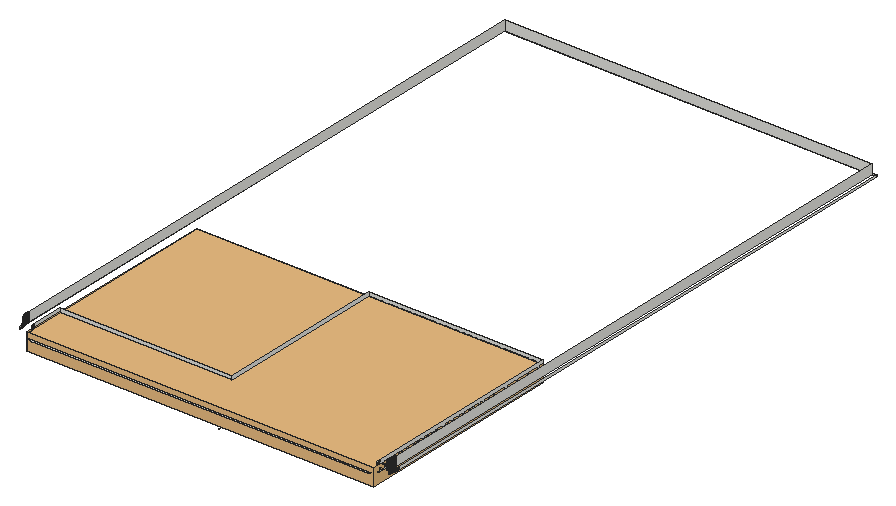
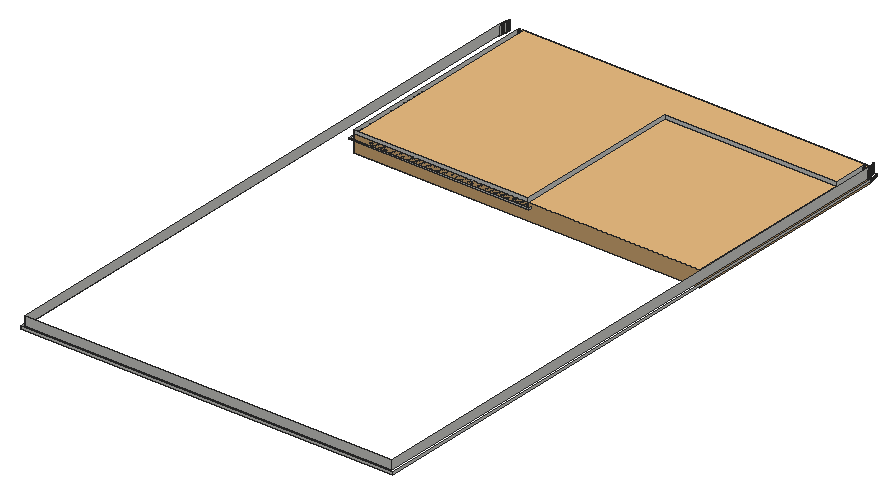
# SketchUp Ruby script. Lengths in inches.
U = 1.inch
M = Sketchup.active_model
def pt(a) = Geom::Point3d.new(a.map { |v| v * U })
def face(e, loops, mat)
  f = e.add_face(loops[0].map { |a| pt(a) })
  loops[1..].each { |l| e.add_face(l.map { |a| pt(a) }).erase! }
  f.material = f.back_material = mat if mat
  f
end
# faces: each face lists its corners as indices into pts; further lists are holes
def faces(e, pts, list, mat = nil) = list.each { |f| face(e, (f[0].is_a?(Array) ? f : [f]).map { |l| l.map { |i| pts[i] } }, mat) }
# xy, xz, yz: faces in a plane at the given z, y or x. An outline is a flat list of corners, or four numbers for a rectangle; further outlines are holes
def ring(l) = l.size == 4 ? [[l[0], l[1]], [l[2], l[1]], [l[2], l[3]], [l[0], l[3]]] : l.each_slice(2).to_a
def flat(e, list, mat, &to3) = list.each { |f| face(e, (f[0].is_a?(Array) ? f : [f]).map { |l| ring(l).map { |u, v| to3.(u, v) } }, mat) }
def xy(e, z, list, mat = nil) = flat(e, list, mat) { |x, y| [x, y, z] }
def xz(e, y, list, mat = nil) = flat(e, list, mat) { |x, z| [x, y, z] }
def yz(e, x, list, mat = nil) = flat(e, list, mat) { |y, z| [x, y, z] }
def lines(e, pts, list) = list.each { |a, b| e.add_line(pt(pts[a]), pt(pts[b])) }
# prism: a flat outline (further loops are holes) pulled along v
def prism(e, loops, v, mat = nil)
  f = face(e, loops, mat); d = Geom::Vector3d.new(v.map { |x| x * U })
  f.pushpull(f.normal.samedirection?(d) ? d.length : -d.length)
end
def box(e, o, s, mat = nil) = prism(e, [[o, [o[0] + s[0], o[1], o[2]], [o[0] + s[0], o[1] + s[1], o[2]], [o[0], o[1] + s[1], o[2]]]], [0, 0, s[2]], mat)
def at(x, y, z, deg = 0) = Geom::Transformation.translation(pt([x, y, z])) * Geom::Transformation.rotation(ORIGIN, Z_AXIS, deg.degrees)
def axes(o, x, y, z) = Geom::Transformation.new([*x, 0, *y, 0, *z, 0, *pt(o).to_a, 1])
def part(name) = M.definitions.add(name)
# library, detail: a bought-in or finely detailed component or shape, given as its bounding box
def library(name, o, s) = part(name).tap { |d| box(d.entities, o, s) }
def detail(e, o, s) = box(e.add_group.entities, o, s)
def put(e, d, t, mat = nil) = e.add_instance(d, t).tap { |i| i.material = mat if mat }
def group(e, t, mat = nil) = e.add_group.tap { |g| g.transformation = t; g.material = mat if mat }.entities
root = M.entities
M.materials.add("Material \#1").color = [140, 140, 140]
c1 = library("Group\#25",[0,0,-11.0625],[292.45,179,14.0625])
xy(root,75.82,[[138.95,197.84,138.95,197.86,138.89,197.86],[138.95,197.84,139.01,197.84,139.01,197.86],[138.95,197.84,139.01,197.86,138.95,197.86],[139.01,197.84,139.0625,197.88,139.01,197.86],[139.01,197.84,139.07,197.86,139.0625,197.88],
  [138.89,197.86,138.9,197.88,138.84,197.9],[138.89,197.86,138.95,197.86,138.9,197.88],[139.07,197.86,139.1,197.91,139.0625,197.88],[139.07,197.86,139.12,197.9,139.1,197.91],[138.9,197.88,138.86,197.91,138.84,197.9],
  [138.84,197.9,138.86,197.91,138.81,197.95],[139.12,197.9,139.13,197.96,139.1,197.91],[139.12,197.9,139.15,197.95,139.13,197.96],[138.86,197.91,138.83,197.96,138.81,197.95],[138.81,197.95,138.83,197.96,138.8,198.01],
  [139.15,197.95,139.14,198.01,139.13,197.96],[139.15,197.95,139.16,198.01,139.14,198.01],[138.83,197.96,138.82,198.01,138.8,198.01],[138.8,198.01,138.82,198.01,138.81,198.07],[138.82,198.01,138.83,198.0625,138.81,198.07],
  [139.14,198.01,139.16,198.01,139.13,198.0625],[139.16,198.01,139.15,198.07,139.13,198.0625],[138.83,198.0625,138.84,198.12,138.81,198.07],[138.83,198.0625,138.86,198.11,138.84,198.12],[139.13,198.0625,139.15,198.07,139.1,198.11],
  [139.15,198.07,139.12,198.12,139.1,198.11],[138.86,198.11,138.89,198.15,138.84,198.12],[138.86,198.11,138.9,198.14,138.89,198.15],[139.1,198.11,139.12,198.12,139.0625,198.14],[139.12,198.12,139.07,198.15,139.0625,198.14],
  [138.9,198.14,138.95,198.17,138.89,198.15],[138.9,198.14,138.95,198.16,138.95,198.17],[139.0625,198.14,139.07,198.15,139.01,198.16],[139.07,198.15,139.01,198.17,139.01,198.16],[138.95,198.16,139.01,198.16,139.01,198.17],
  [138.95,198.16,139.01,198.17,138.95,198.17]],"Material \#1")
xy(root,75.84,[[138.95,197.84,138.89,197.86,138.9,197.88],[138.95,197.84,138.9,197.88,138.95,197.86],[138.95,197.84,138.95,197.86,139.01,197.84],[139.01,197.84,138.95,197.86,139.01,197.86],[139.01,197.84,139.01,197.86,139.07,197.86],
  [138.89,197.86,138.84,197.9,138.86,197.91],[138.89,197.86,138.86,197.91,138.9,197.88],[139.01,197.86,139.0625,197.88,139.07,197.86],[139.07,197.86,139.0625,197.88,139.12,197.9],[139.0625,197.88,139.1,197.91,139.12,197.9],
  [138.84,197.9,138.81,197.95,138.83,197.96],[138.84,197.9,138.83,197.96,138.86,197.91],[139.12,197.9,139.1,197.91,139.15,197.95],[139.1,197.91,139.13,197.96,139.15,197.95],[138.81,197.95,138.8,198.01,138.82,198.01],
  [138.81,197.95,138.82,198.01,138.83,197.96],[139.15,197.95,139.13,197.96,139.16,198.01],[139.13,197.96,139.14,198.01,139.16,198.01],[138.8,198.01,138.81,198.07,138.83,198.0625],[138.8,198.01,138.83,198.0625,138.82,198.01],
  [139.14,198.01,139.13,198.0625,139.15,198.07],[139.14,198.01,139.15,198.07,139.16,198.01],[138.83,198.0625,138.81,198.07,138.86,198.11],[139.13,198.0625,139.1,198.11,139.12,198.12],[139.13,198.0625,139.12,198.12,139.15,198.07],
  [138.81,198.07,138.84,198.12,138.86,198.11],[138.86,198.11,138.84,198.12,138.9,198.14],[139.1,198.11,139.0625,198.14,139.07,198.15],[139.1,198.11,139.07,198.15,139.12,198.12],[138.84,198.12,138.89,198.15,138.9,198.14],
  [138.9,198.14,138.89,198.15,138.95,198.16],[139.0625,198.14,139.01,198.16,139.01,198.17],[139.0625,198.14,139.01,198.17,139.07,198.15],[138.89,198.15,138.95,198.17,138.95,198.16],[138.95,198.16,138.95,198.17,139.01,198.16],
  [139.01,198.16,138.95,198.17,139.01,198.17]],"Material \#1")
xy(root,79.36,[[138.95,197.84,138.9,197.88,138.89,197.86],[138.95,197.84,138.95,197.86,138.9,197.88],[138.95,197.84,139.01,197.84,138.95,197.86],[139.01,197.84,139.01,197.86,138.95,197.86],[139.01,197.84,139.07,197.86,139.01,197.86],
  [138.89,197.86,138.86,197.91,138.84,197.9],[138.89,197.86,138.9,197.88,138.86,197.91],[139.01,197.86,139.07,197.86,139.0625,197.88],[139.07,197.86,139.12,197.9,139.0625,197.88],[139.0625,197.88,139.12,197.9,139.1,197.91],
  [138.84,197.9,138.83,197.96,138.81,197.95],[138.84,197.9,138.86,197.91,138.83,197.96],[139.12,197.9,139.15,197.95,139.1,197.91],[139.1,197.91,139.15,197.95,139.13,197.96],[138.81,197.95,138.82,198.01,138.8,198.01],
  [138.81,197.95,138.83,197.96,138.82,198.01],[139.15,197.95,139.16,198.01,139.13,197.96],[139.13,197.96,139.16,198.01,139.14,198.01],[138.8,198.01,138.82,198.01,138.83,198.0625],[138.8,198.01,138.83,198.0625,138.81,198.07],
  [139.14,198.01,139.15,198.07,139.13,198.0625],[139.14,198.01,139.16,198.01,139.15,198.07],[138.83,198.0625,138.86,198.11,138.81,198.07],[139.13,198.0625,139.12,198.12,139.1,198.11],[139.13,198.0625,139.15,198.07,139.12,198.12],
  [138.81,198.07,138.86,198.11,138.84,198.12],[138.86,198.11,138.9,198.14,138.84,198.12],[139.1,198.11,139.07,198.15,139.0625,198.14],[139.1,198.11,139.12,198.12,139.07,198.15],[138.84,198.12,138.9,198.14,138.89,198.15],
  [138.9,198.14,138.95,198.16,138.89,198.15],[139.0625,198.14,139.01,198.17,139.01,198.16],[139.0625,198.14,139.07,198.15,139.01,198.17],[138.89,198.15,138.95,198.16,138.95,198.17],[138.95,198.16,139.01,198.16,138.95,198.17],
  [139.01,198.16,139.01,198.17,138.95,198.17]],"Material \#1")
xy(root,79.375,[[138.95,197.84,138.89,197.86,138.95,197.86],[138.95,197.84,138.95,197.86,139.01,197.86],[138.95,197.84,139.01,197.86,139.01,197.84],[139.01,197.84,139.01,197.86,139.0625,197.88],[139.01,197.84,139.0625,197.88,139.07,197.86],
  [138.89,197.86,138.84,197.9,138.9,197.88],[138.89,197.86,138.9,197.88,138.95,197.86],[139.07,197.86,139.0625,197.88,139.1,197.91],[139.07,197.86,139.1,197.91,139.12,197.9],[138.9,197.88,138.84,197.9,138.86,197.91],
  [138.84,197.9,138.81,197.95,138.86,197.91],[139.12,197.9,139.1,197.91,139.13,197.96],[139.12,197.9,139.13,197.96,139.15,197.95],[138.86,197.91,138.81,197.95,138.83,197.96],[138.81,197.95,138.8,198.01,138.83,197.96],
  [139.15,197.95,139.13,197.96,139.14,198.01],[139.15,197.95,139.14,198.01,139.16,198.01],[138.83,197.96,138.8,198.01,138.82,198.01],[138.8,198.01,138.81,198.07,138.82,198.01],[138.82,198.01,138.81,198.07,138.83,198.0625],
  [139.14,198.01,139.13,198.0625,139.16,198.01],[139.16,198.01,139.13,198.0625,139.15,198.07],[138.83,198.0625,138.81,198.07,138.84,198.12],[138.83,198.0625,138.84,198.12,138.86,198.11],[139.13,198.0625,139.1,198.11,139.15,198.07],
  [139.15,198.07,139.1,198.11,139.12,198.12],[138.86,198.11,138.84,198.12,138.89,198.15],[138.86,198.11,138.89,198.15,138.9,198.14],[139.1,198.11,139.0625,198.14,139.12,198.12],[139.12,198.12,139.0625,198.14,139.07,198.15],
  [138.9,198.14,138.89,198.15,138.95,198.17],[138.9,198.14,138.95,198.17,138.95,198.16],[139.0625,198.14,139.01,198.16,139.07,198.15],[139.07,198.15,139.01,198.16,139.01,198.17],[138.95,198.16,138.95,198.17,139.01,198.17],
  [138.95,198.16,139.01,198.17,139.01,198.16]],"Material \#1")
xy(root,119,[[[17.82,153,17.65,153.01,17.29,153.03,17.12,153.04,16.94,153.0625,16.77,153.08,16.59,153.11,16.42,153.14,16.24,153.17,15.73,153.29,15.22,153.44,14.88,153.56,14.72,153.62,14.56,153.69,14.39,153.75,14.23,153.83,14.07,153.9,13.91,153.98,13.76,154.0625,13.6,154.15,13.15,154.42,12.85,154.62,12.57,154.82,12.29,155.04,12.15,155.16,12.02,155.27,11.76,155.51,11.64,155.64,11.51,155.76,11.27,156.02,11.16,156.15,11.04,156.29,10.82,156.57,10.62,156.85,10.42,157.15,10.15,157.6,10.0625,157.76,9.98,157.91,9.9,158.07,9.83,158.23,9.75,158.39,9.69,158.56,9.62,158.72,9.56,158.88,9.44,159.22,9.29,159.73,9.17,160.24,9.14,160.42,9.11,160.59,9.08,160.77,9.0625,160.94,9.04,161.12,9.03,161.29,9.01,161.65,9,161.82,9,192,154.05,192,154.05,336,305.45,336,305.45,162,305.375,160.83,305.15,159.67,304.77,158.56,304.25,157.5,303.59,156.52,302.82,155.64,301.93,154.86,300.95,154.21,299.9,153.69,298.78,153.31,297.63,153.08,296.45,153],[17.86,155,296.45,155,297.37,155.06,298.27,155.24,299.13,155.53,299.95,155.9375,300.71,156.45,301.4,157.05,302.01,157.74,302.52,158.5,302.92,159.32,303.21,160.1875,303.39,161.09,303.45,162,303.45,334,156.05,334,156.05,190,11,190,11,161.86,11.01,161.73,11.01,161.59,11.02,161.45,11.03,161.3125,11.05,161.18,11.09,160.9,11.11,160.77,11.13,160.63,11.19,160.37,11.23,160.23,11.26,160.1,11.34,159.84,11.39,159.71,11.43,159.58,11.53,159.32,11.59,159.19,11.64,159.07,11.7,158.95,11.76,158.82,11.83,158.7,11.89,158.58,12.03,158.34,12.1,158.23,12.18,158.11,12.5,157.67,12.68,157.45,12.95,157.15,13.15,156.95,13.45,156.68,13.67,156.5,14.11,156.18,14.23,156.1,14.34,156.03,14.58,155.89,14.7,155.83,14.82,155.76,14.95,155.7,15.07,155.64,15.19,155.59,15.32,155.53,15.58,155.43,15.71,155.39,15.84,155.34,16.1,155.26,16.23,155.23,16.37,155.19,16.63,155.13,16.77,155.11,16.9,155.09,17.18,155.05,17.3125,155.03,17.45,155.02,17.59,155.01,17.73,155.01]]])
xz(root,190,[[11,119,156.05,126]])
xz(root,192,[[9,119,154.05,120]])
xz(root,334,[[156.05,119,303.45,126]])
xz(root,336,[[154.05,119,305.45,120]])
xz(root,670,[[2.02,122,312.4375,130]])
xz(root,672,[[0,120,314.45,122]])
yz(root,0,[[167.6875,120,168,122],[168,120,672,122]])
yz(root,2.02,[[167.42,122,167.71,130],[167.71,122,168,130],[168,122,670,130]])
yz(root,9,[[161.82,119,162,120],[162,119,192,120]])
yz(root,11,[[161.86,119,162,126],[162,119,190,126]])
yz(root,11.01,[[161.59,119,161.73,126]])
yz(root,154.05,[[192,119,336,120]])
yz(root,156.05,[[190,119,334,126]])
yz(root,303.45,[[162,119,334,126]])
yz(root,305.45,[[162,119,336,120]])
yz(root,312.4375,[[167.71,122,168,130],[168,122,670,130]])
yz(root,314.45,[[167.37,120,167.6875,122],[167.6875,120,168,122],[168,120,672,122]])
p = [[302.92,159.32,126],[303.21,160.1875,126],[303.21,160.1875,119],[302.92,159.32,119],[9.34,159.56,120],[9.29,159.73,120],
  [9.29,159.73,119],[9.34,159.56,119],[11.39,159.71,126],[11.43,159.58,126],[11.43,159.58,119],[11.39,159.71,119],
  [9.25,159.9,120],[9.25,159.9,119],[11.34,159.84,126],[11.34,159.84,119],[305.375,160.83,120],[305.15,159.67,120],
  [305.15,159.67,119],[305.375,160.83,119],[11.3,159.97,126],[11.3,159.97,119],[9.21,160.07,120],[9.21,160.07,119],
  [11.26,160.1,126],[11.26,160.1,119],[9.17,160.24,120],[9.17,160.24,119],[11.23,160.23,126],[11.23,160.23,119],
  [9.14,160.42,120],[9.14,160.42,119],[11.19,160.37,126],[11.19,160.37,119],[303.39,161.09,126],[303.39,161.09,119],
  [9.11,160.59,120],[9.11,160.59,119],[11.16,160.5,126],[11.16,160.5,119],[11.13,160.63,126],[11.13,160.63,119],
  [9.08,160.77,120],[9.08,160.77,119],[11.11,160.77,126],[11.11,160.77,119],[9.0625,160.94,120],[9.0625,160.94,119],
  [11.09,160.9,126],[11.09,160.9,119],[305.45,162,120],[305.45,162,119],[9.04,161.12,120],[9.04,161.12,119],
  [11.07,161.04,126],[11.07,161.04,119],[11.05,161.18,126],[11.05,161.18,119],[9.03,161.29,120],[9.03,161.29,119],
  [303.45,162,126],[303.45,162,119],[11.03,161.3125,126],[11.03,161.3125,119],[9.02,161.47,120],[9.02,161.47,119],
  [11.02,161.45,126],[11.02,161.45,119],[9.01,161.65,120],[9.01,161.65,119],[11.01,161.59,126],[11.01,161.59,119],
  [9,161.82,120],[9,161.82,119],[11,161.86,126],[11.01,161.73,126],[11.01,161.73,119],[11,161.86,119],
  [1.39,159.99,120],[1.5,159.69,120],[1.5,159.69,122],[1.39,159.99,122],[312.96,159.69,120],[313.07,159.99,120],
  [313.07,159.99,122],[312.96,159.69,122],[1.28,160.29,120],[1.28,160.29,122],[313.17,160.29,120],[313.17,160.29,122],
  [1.18,160.58,120],[1.18,160.58,122],[313.27,160.58,120],[313.27,160.58,122],[1.09,160.88,120],[1.09,160.88,122],
  [313.37,160.88,120],[313.37,160.88,122],[1,161.18,120],[1,161.18,122],[313.46,161.18,120],[313.46,161.18,122],
  [0.91,161.49,120],[0.91,161.49,122],[313.55,161.49,120],[313.55,161.49,122],[0.82,161.79,120],[0.82,161.79,122],
  [313.63,161.79,120],[313.63,161.79,122],[0.74,162.09,120],[0.74,162.09,122],[313.71,162.09,120],[313.71,162.09,122],
  [0.67,162.4,120],[0.67,162.4,122],[313.79,162.4,120],[313.79,162.4,122],[0.6,162.7,120],[0.6,162.7,122],
  [313.86,162.7,120],[313.86,162.7,122],[0.53,163.01,120],[0.53,163.01,122],[313.92,163.01,120],[313.92,163.01,122],
  [0.46,163.32,120],[0.46,163.32,122],[313.99,163.32,120],[313.99,163.32,122],[0.41,163.625,120],[0.41,163.625,122],
  [314.05,163.625,120],[314.05,163.625,122],[0.35,163.9375,120],[0.35,163.9375,122],[314.1,163.9375,120],[314.1,163.9375,122],
  [0.3,164.25,120],[0.3,164.25,122],[314.16,164.25,120],[314.16,164.25,122],[0.25,164.56,120],[0.25,164.56,122],
  [314.2,164.56,120],[314.2,164.56,122],[0.21,164.87,120],[0.21,164.87,122],[314.25,164.87,120],[314.25,164.87,122],
  [0.17,165.18,120],[0.17,165.18,122],[314.29,165.18,120],[314.29,165.18,122],[0.13,165.49,120],[0.13,165.49,122],
  [314.32,165.49,120],[314.32,165.49,122],[0.1,165.8,120],[0.1,165.8,122],[314.35,165.8,120],[314.35,165.8,122],
  [0.07,166.12,120],[0.07,166.12,122],[314.38,166.12,120],[314.38,166.12,122],[0.05,166.43,120],[0.05,166.43,122],
  [314.4,166.43,120],[314.4,166.43,122],[0.03,166.74,120],[0.03,166.74,122],[314.42,166.74,120],[314.42,166.74,122],
  [0.02,167.06,120],[0.02,167.06,122],[314.43,167.06,120],[314.43,167.06,122],[0.01,167.37,120],[0.01,167.37,122],
  [314.45,167.37,120],[314.45,167.37,122],[0,167.6875,120],[0,167.6875,122],[3.59,159.85,122],[3.7,159.58,122],
  [3.7,159.58,130],[3.59,159.85,130],[310.75,159.58,122],[310.86,159.85,122],[310.86,159.85,130],[310.75,159.58,130],
  [3.49,160.12,122],[3.49,160.12,130],[310.96,160.12,122],[310.96,160.12,130],[3.39,160.39,122],[3.39,160.39,130],
  [311.07,160.39,122],[311.07,160.39,130],[3.29,160.66,122],[3.29,160.66,130],[311.17,160.66,122],[311.17,160.66,130],
  [3.19,160.93,122],[3.19,160.93,130],[311.26,160.93,122],[311.26,160.93,130],[3.1,161.2,122],[3.1,161.2,130],
  [311.35,161.2,122],[311.35,161.2,130],[3.01,161.48,122],[3.01,161.48,130],[311.44,161.48,122],[311.44,161.48,130],
  [2.93,161.75,122],[2.93,161.75,130],[311.52,161.75,122],[311.52,161.75,130],[2.85,162.03,122],[2.85,162.03,130],
  [311.61,162.03,122],[311.61,162.03,130],[2.77,162.31,122],[2.77,162.31,130],[311.68,162.31,122],[311.68,162.31,130],
  [2.7,162.58,122],[2.7,162.58,130],[311.76,162.58,122],[311.76,162.58,130],[2.63,162.86,122],[2.63,162.86,130],
  [311.83,162.86,122],[311.83,162.86,130],[2.5625,163.14,122],[2.5625,163.14,130],[311.89,163.14,122],[311.89,163.14,130],
  [2.5,163.43,122],[2.5,163.43,130],[311.95,163.43,122],[311.95,163.43,130],[2.44,163.71,122],[2.44,163.71,130],
  [312.01,163.71,122],[312.01,163.71,130],[2.39,163.99,122],[2.39,163.99,130],[312.07,163.99,122],[312.07,163.99,130],
  [2.34,164.27,122],[2.34,164.27,130],[312.12,164.27,122],[312.12,164.27,130],[2.29,164.56,122],[2.29,164.56,130],
  [312.16,164.56,122],[312.16,164.56,130],[2.25,164.84,122],[2.25,164.84,130],[312.21,164.84,122],[312.21,164.84,130],
  [2.21,165.13,122],[2.21,165.13,130],[312.25,165.13,122],[312.25,165.13,130],[2.17,165.41,122],[2.17,165.41,130],
  [312.28,165.41,122],[312.28,165.41,130],[2.14,165.7,122],[2.14,165.7,130],[312.32,165.7,122],[312.32,165.7,130],
  [2.11,165.99,122],[2.11,165.99,130],[312.34,165.99,122],[312.34,165.99,130],[2.08,166.27,122],[2.08,166.27,130],
  [312.37,166.27,122],[312.37,166.27,130],[2.0625,166.5625,122],[2.0625,166.5625,130],[312.39,166.5625,122],[312.39,166.5625,130],
  [2.05,166.85,122],[2.05,166.85,130],[312.41,166.85,122],[312.41,166.85,130],[2.03,167.14,122],[2.03,167.14,130],
  [312.42,167.14,122],[312.42,167.14,130],[2.02,167.42,122],[2.02,167.42,130],[312.43,167.42,122],[312.43,167.42,130],
  [312.4375,167.71,122],[312.4375,167.71,130]]
faces(root,p,[[0,1,2,3],[4,5,6,7],[8,9,10,11],[5,12,13,6],[14,8,11,15],[16,17,18,19],[20,14,15,21],[12,22,23,13],
  [24,20,21,25],[22,26,27,23],[28,24,25,29],[26,30,31,27],[32,28,29,33],[1,34,35,2],[30,36,37,31],[38,32,33,39],
  [40,38,39,41],[36,42,43,37],[44,40,41,45],[42,46,47,43],[48,44,45,49],[50,16,19,51],[46,52,53,47],[54,48,49,55],
  [56,54,55,57],[52,58,59,53],[34,60,61,35],[62,56,57,63],[58,64,65,59],[66,62,63,67],[64,68,69,65],[70,66,67,71],
  [68,72,73,69],[74,75,76,77],[78,79,80,81],[82,83,84,85],[86,78,81,87],[83,88,89,84],[90,86,87,91],[88,92,93,89],
  [94,90,91,95],[92,96,97,93],[98,94,95,99],[96,100,101,97],[102,98,99,103],[100,104,105,101],[106,102,103,107],[104,108,109,105],
  [110,106,107,111],[108,112,113,109],[114,110,111,115],[112,116,117,113],[118,114,115,119],[116,120,121,117],[122,118,119,123],[120,124,125,121],
  [126,122,123,127],[124,128,129,125],[130,126,127,131],[128,132,133,129],[134,130,131,135],[132,136,137,133],[138,134,135,139],[136,140,141,137],
  [142,138,139,143],[140,144,145,141],[146,142,143,147],[144,148,149,145],[150,146,147,151],[148,152,153,149],[154,150,151,155],[152,156,157,153],
  [158,154,155,159],[156,160,161,157],[162,158,159,163],[160,164,165,161],[166,162,163,167],[164,168,169,165],[170,166,167,171],[168,172,173,169],
  [174,170,171,175],[172,176,177,173],[178,174,175,179],[176,180,181,177],[182,178,179,183],[184,185,186,187],[188,189,190,191],[192,184,187,193],
  [189,194,195,190],[196,192,193,197],[194,198,199,195],[200,196,197,201],[198,202,203,199],[204,200,201,205],[202,206,207,203],[208,204,205,209],
  [206,210,211,207],[212,208,209,213],[210,214,215,211],[216,212,213,217],[214,218,219,215],[220,216,217,221],[218,222,223,219],[224,220,221,225],
  [222,226,227,223],[228,224,225,229],[226,230,231,227],[232,228,229,233],[230,234,235,231],[236,232,233,237],[234,238,239,235],[240,236,237,241],
  [238,242,243,239],[244,240,241,245],[242,246,247,243],[248,244,245,249],[246,250,251,247],[252,248,249,253],[250,254,255,251],[256,252,253,257],
  [254,258,259,255],[260,256,257,261],[258,262,263,259],[264,260,261,265],[262,266,267,263],[268,264,265,269],[266,270,271,267],[272,268,269,273],
  [270,274,275,271],[276,272,273,277],[274,278,279,275],[280,276,277,281],[278,282,283,279],[284,280,281,285],[282,286,287,283],[288,284,285,289],
  [286,290,291,287],[292,288,289,293],[290,294,295,291],[296,292,293,297],[294,298,299,295],[298,300,301,299]])
put(root,c1,at(11,155,120))
